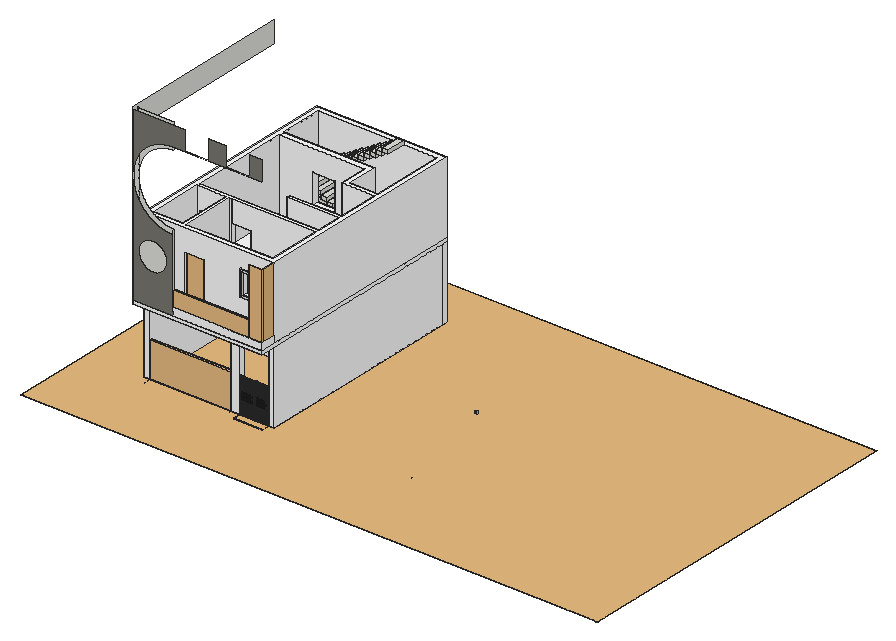
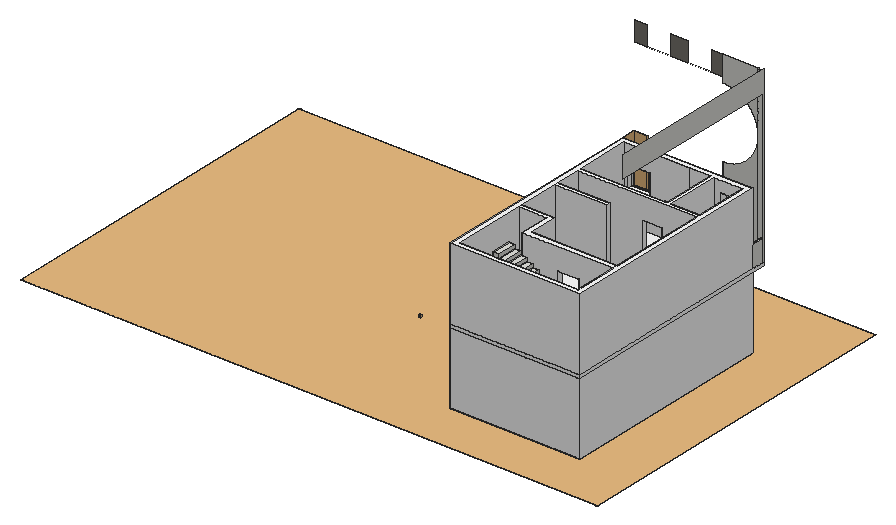
# SketchUp Ruby script. Lengths in inches.
U = 1.inch
M = Sketchup.active_model
def pt(a) = Geom::Point3d.new(a.map { |v| v * U })
def face(e, loops, mat)
  f = e.add_face(loops[0].map { |a| pt(a) })
  loops[1..].each { |l| e.add_face(l.map { |a| pt(a) }).erase! }
  f.material = f.back_material = mat if mat
  f
end
# faces: each face lists its corners as indices into pts; further lists are holes
def faces(e, pts, list, mat = nil) = list.each { |f| face(e, (f[0].is_a?(Array) ? f : [f]).map { |l| l.map { |i| pts[i] } }, mat) }
# xy, xz, yz: faces in a plane at the given z, y or x. An outline is a flat list of corners, or four numbers for a rectangle; further outlines are holes
def ring(l) = l.size == 4 ? [[l[0], l[1]], [l[2], l[1]], [l[2], l[3]], [l[0], l[3]]] : l.each_slice(2).to_a
def flat(e, list, mat, &to3) = list.each { |f| face(e, (f[0].is_a?(Array) ? f : [f]).map { |l| ring(l).map { |u, v| to3.(u, v) } }, mat) }
def xy(e, z, list, mat = nil) = flat(e, list, mat) { |x, y| [x, y, z] }
def xz(e, y, list, mat = nil) = flat(e, list, mat) { |x, z| [x, y, z] }
def yz(e, x, list, mat = nil) = flat(e, list, mat) { |y, z| [x, y, z] }
def lines(e, pts, list) = list.each { |a, b| e.add_line(pt(pts[a]), pt(pts[b])) }
# prism: a flat outline (further loops are holes) pulled along v
def prism(e, loops, v, mat = nil)
  f = face(e, loops, mat); d = Geom::Vector3d.new(v.map { |x| x * U })
  f.pushpull(f.normal.samedirection?(d) ? d.length : -d.length)
end
def box(e, o, s, mat = nil) = prism(e, [[o, [o[0] + s[0], o[1], o[2]], [o[0] + s[0], o[1] + s[1], o[2]], [o[0], o[1] + s[1], o[2]]]], [0, 0, s[2]], mat)
def at(x, y, z, deg = 0) = Geom::Transformation.translation(pt([x, y, z])) * Geom::Transformation.rotation(ORIGIN, Z_AXIS, deg.degrees)
def axes(o, x, y, z) = Geom::Transformation.new([*x, 0, *y, 0, *z, 0, *pt(o).to_a, 1])
def part(name) = M.definitions.add(name)
# library, detail: a bought-in or finely detailed component or shape, given as its bounding box
def library(name, o, s) = part(name).tap { |d| box(d.entities, o, s) }
def detail(e, o, s) = box(e.add_group.entities, o, s)
def put(e, d, t, mat = nil) = e.add_instance(d, t).tap { |i| i.material = mat if mat }
def group(e, t, mat = nil) = e.add_group.tap { |g| g.transformation = t; g.material = mat if mat }.entities
root = M.entities
M.materials.add("Color_008").color = [30, 30, 30]
M.materials.add("Manhattan Creative Coating ML 1016B 24.75cm").color = [255, 255, 255]
M.materials.add("Napura - nsi3013 29.32cm").color = [255, 255, 255]
M.materials.add("Sand Yellow 02 100cm").color = [219, 192, 169]
M.materials.add("Tiles L02 200cm").color = [152, 144, 134]
M.materials.add("[0055_LightGoldenrodYellow]").color = [250, 250, 210]
M.materials.add("[0131_Silver]").color = [192, 192, 192]
M.materials.add("[0134_DimGray]").color = [105, 105, 105]
M.materials.add("[Rough Square Concrete Block]").color = [123, 120, 113]
c1 = library("Garage Gate 243 111",[-105.76,-3.7,0],[211.52,7.4,101.23])
c2 = part("Screen slat")
box(c2.entities,[0,0,-2.03],[1.97,0.97,40.94])
c3 = part("Screen frame stile")
box(c3.entities,[0,0,0],[1.9,0.97,93.54])
c4 = part("Screen bar")
box(c4.entities,[2.95,0,-2.03],[0.99,0.97,40.94])
c5 = part("Slatted screen panel")
p = [[42.85,0.97,43.31],[42.85,0.97,44.29]]
lines(c5.entities,p,[[0,1]])
put(c5.entities,c2,axes([3.9375,0,86.61],[0,0,-1],[0,1,0],[1,0,0]),"Color_008")
put(c5.entities,c3,axes([87.6,0,0],[1,0,0],[0,1,0],[0,0,0.92593]),"Color_008")
put(c5.entities,c2,axes([48.6875,0,86.61],[0,0,-1],[0,1,0],[1,0,0]),"Color_008")
put(c5.entities,c3,axes([0,0,0],[1,0,0],[0,1,0],[0,0,0.92593]),"Color_008")
put(c5.entities,c3,axes([42.85,0,0],[1,0,0],[0,1,0],[0,0,0.92593]),"Color_008")
put(c5.entities,c3,axes([44.75,0,0],[1,0,0],[0,1,0],[0,0,0.92593]),"Color_008")
put(c5.entities,c4,axes([3.9375,0,87.11],[0,0,-1],[0,1,0],[1,0,0]),"[0134_DimGray]")
put(c5.entities,c4,axes([48.6875,0,87.11],[0,0,-1],[0,1,0],[1,0,0]),"[0134_DimGray]")
put(c5.entities,c2,axes([48.6875,0,82.68],[0,0,-1],[0,1,0],[1,0,0]),"Color_008")
put(c5.entities,c4,axes([48.6875,0,83.17],[0,0,-1],[0,1,0],[1,0,0]),"[0134_DimGray]")
put(c5.entities,c4,axes([3.9375,0,83.17],[0,0,-1],[0,1,0],[1,0,0]),"[0134_DimGray]")
put(c5.entities,c2,axes([3.9375,0,82.68],[0,0,-1],[0,1,0],[1,0,0]),"Color_008")
put(c5.entities,c4,axes([48.6875,0,75.3],[0,0,-1],[0,1,0],[1,0,0]),"[0134_DimGray]")
put(c5.entities,c2,axes([48.6875,0,78.74],[0,0,-1],[0,1,0],[1,0,0]),"Color_008")
put(c5.entities,c2,axes([48.6875,0,74.8],[0,0,-1],[0,1,0],[1,0,0]),"Color_008")
put(c5.entities,c4,axes([48.6875,0,79.23],[0,0,-1],[0,1,0],[1,0,0]),"[0134_DimGray]")
put(c5.entities,c4,axes([3.9375,0,75.3],[0,0,-1],[0,1,0],[1,0,0]),"[0134_DimGray]")
put(c5.entities,c2,axes([3.9375,0,78.74],[0,0,-1],[0,1,0],[1,0,0]),"Color_008")
put(c5.entities,c4,axes([3.9375,0,79.23],[0,0,-1],[0,1,0],[1,0,0]),"[0134_DimGray]")
put(c5.entities,c2,axes([3.9375,0,74.8],[0,0,-1],[0,1,0],[1,0,0]),"Color_008")
put(c5.entities,c4,axes([48.6875,0,67.42],[0,0,-1],[0,1,0],[1,0,0]),"[0134_DimGray]")
put(c5.entities,c4,axes([3.9375,0,63.48],[0,0,-1],[0,1,0],[1,0,0]),"[0134_DimGray]")
put(c5.entities,c4,axes([48.6875,0,71.36],[0,0,-1],[0,1,0],[1,0,0]),"[0134_DimGray]")
put(c5.entities,c4,axes([3.9375,0,67.42],[0,0,-1],[0,1,0],[1,0,0]),"[0134_DimGray]")
put(c5.entities,c2,axes([3.9375,0,70.87],[0,0,-1],[0,1,0],[1,0,0]),"Color_008")
put(c5.entities,c2,axes([48.6875,0,70.87],[0,0,-1],[0,1,0],[1,0,0]),"Color_008")
put(c5.entities,c2,axes([48.6875,0,66.93],[0,0,-1],[0,1,0],[1,0,0]),"Color_008")
put(c5.entities,c2,axes([48.6875,0,59.06],[0,0,-1],[0,1,0],[1,0,0]),"Color_008")
put(c5.entities,c2,axes([3.9375,0,55.12],[0,0,-1],[0,1,0],[1,0,0]),"Color_008")
put(c5.entities,c2,axes([3.9375,0,62.99],[0,0,-1],[0,1,0],[1,0,0]),"Color_008")
put(c5.entities,c4,axes([3.9375,0,59.55],[0,0,-1],[0,1,0],[1,0,0]),"[0134_DimGray]")
put(c5.entities,c2,axes([3.9375,0,66.93],[0,0,-1],[0,1,0],[1,0,0]),"Color_008")
put(c5.entities,c2,axes([48.6875,0,62.99],[0,0,-1],[0,1,0],[1,0,0]),"Color_008")
put(c5.entities,c4,axes([48.6875,0,59.55],[0,0,-1],[0,1,0],[1,0,0]),"[0134_DimGray]")
put(c5.entities,c4,axes([48.6875,0,63.48],[0,0,-1],[0,1,0],[1,0,0]),"[0134_DimGray]")
put(c5.entities,c2,axes([3.9375,0,59.06],[0,0,-1],[0,1,0],[1,0,0]),"Color_008")
put(c5.entities,c4,axes([3.9375,0,71.36],[0,0,-1],[0,1,0],[1,0,0]),"[0134_DimGray]")
put(c5.entities,c4,axes([3.9375,0,33.96],[0,0,-1],[0,1,0],[1,0,0]),"[0134_DimGray]")
put(c5.entities,c4,axes([48.6875,0,33.96],[0,0,-1],[0,1,0],[1,0,0]),"[0134_DimGray]")
put(c5.entities,c2,axes([3.9375,0,29.53],[0,0,-1],[0,1,0],[1,0,0]),"Color_008")
put(c5.entities,c4,axes([3.9375,0,26.08],[0,0,-1],[0,1,0],[1,0,0]),"[0134_DimGray]")
put(c5.entities,c2,axes([3.9375,0,33.46],[0,0,-1],[0,1,0],[1,0,0]),"Color_008")
put(c5.entities,c2,axes([48.6875,0,29.53],[0,0,-1],[0,1,0],[1,0,0]),"Color_008")
put(c5.entities,c4,axes([48.6875,0,30.02],[0,0,-1],[0,1,0],[1,0,0]),"[0134_DimGray]")
put(c5.entities,c2,axes([3.9375,0,25.59],[0,0,-1],[0,1,0],[1,0,0]),"Color_008")
put(c5.entities,c2,axes([48.6875,0,25.59],[0,0,-1],[0,1,0],[1,0,0]),"Color_008")
put(c5.entities,c2,axes([48.6875,0,33.46],[0,0,-1],[0,1,0],[1,0,0]),"Color_008")
put(c5.entities,c2,axes([3.9375,0,49.7],[0,0,-1],[0,1,0],[1,0,0]),"Color_008")
put(c5.entities,c4,axes([48.6875,0,26.08],[0,0,-1],[0,1,0],[1,0,0]),"[0134_DimGray]")
put(c5.entities,c4,axes([3.9375,0,30.02],[0,0,-1],[0,1,0],[1,0,0]),"[0134_DimGray]")
put(c5.entities,c2,axes([3.9375,0,5.91],[0,0,-1],[0,1,0],[1,0,0]),"Color_008")
put(c5.entities,c2,axes([48.6875,0,13.78],[0,0,-1],[0,1,0],[1,0,0]),"Color_008")
put(c5.entities,c4,axes([48.6875,0,10.33],[0,0,-1],[0,1,0],[1,0,0]),"[0134_DimGray]")
put(c5.entities,c4,axes([3.9375,0,6.4],[0,0,-1],[0,1,0],[1,0,0]),"[0134_DimGray]")
put(c5.entities,c2,axes([3.9375,0,13.78],[0,0,-1],[0,1,0],[1,0,0]),"Color_008")
put(c5.entities,c2,axes([48.6875,0,21.65],[0,0,-1],[0,1,0],[1,0,0]),"Color_008")
put(c5.entities,c2,axes([48.6875,0,5.91],[0,0,-1],[0,1,0],[1,0,0]),"Color_008")
put(c5.entities,c4,axes([48.6875,0,22.15],[0,0,-1],[0,1,0],[1,0,0]),"[0134_DimGray]")
put(c5.entities,c2,axes([48.6875,0,1.97],[0,0,-1],[0,1,0],[1,0,0]),"Color_008")
put(c5.entities,c2,axes([48.6875,0,9.84],[0,0,-1],[0,1,0],[1,0,0]),"Color_008")
put(c5.entities,c4,axes([48.6875,0,6.4],[0,0,-1],[0,1,0],[1,0,0]),"[0134_DimGray]")
put(c5.entities,c2,axes([3.9375,0,9.84],[0,0,-1],[0,1,0],[1,0,0]),"Color_008")
put(c5.entities,c4,axes([3.9375,0,10.33],[0,0,-1],[0,1,0],[1,0,0]),"[0134_DimGray]")
put(c5.entities,c4,axes([3.9375,0,22.15],[0,0,-1],[0,1,0],[1,0,0]),"[0134_DimGray]")
put(c5.entities,c2,axes([3.9375,0,1.97],[0,0,-1],[0,1,0],[1,0,0]),"Color_008")
put(c5.entities,c4,axes([3.9375,0,18.21],[0,0,-1],[0,1,0],[1,0,0]),"[0134_DimGray]")
put(c5.entities,c4,axes([3.9375,0,14.27],[0,0,-1],[0,1,0],[1,0,0]),"[0134_DimGray]")
put(c5.entities,c2,axes([3.9375,0,21.65],[0,0,-1],[0,1,0],[1,0,0]),"Color_008")
put(c5.entities,c4,axes([48.6875,0,18.21],[0,0,-1],[0,1,0],[1,0,0]),"[0134_DimGray]")
put(c5.entities,c2,axes([3.9375,0,17.72],[0,0,-1],[0,1,0],[1,0,0]),"Color_008")
put(c5.entities,c2,axes([48.6875,0,17.72],[0,0,-1],[0,1,0],[1,0,0]),"Color_008")
put(c5.entities,c4,axes([48.6875,0,14.27],[0,0,-1],[0,1,0],[1,0,0]),"[0134_DimGray]")
put(c5.entities,c2,axes([3.9375,0,44.29],[0,0,-1],[0,1,0],[1,0,0]),"Color_008")
put(c5.entities,c2,axes([3.9375,0,38.88],[0,0,-1],[0,1,0],[1,0,0]),"Color_008")
put(c5.entities,c2,axes([48.6875,0,49.7],[0,0,-1],[0,1,0],[1,0,0]),"Color_008")
put(c5.entities,c2,axes([48.6875,0,44.29],[0,0,-1],[0,1,0],[1,0,0]),"Color_008")
put(c5.entities,c2,axes([48.6875,0,38.88],[0,0,-1],[0,1,0],[1,0,0]),"Color_008")
put(c5.entities,c2,axes([48.6875,0,55.12],[0,0,-1],[0,1,0],[1,0,0]),"Color_008")
c6 = part("Infill panel")
box(c6.entities,[0,0,-9.84],[39.64,0.39,36.58])
c7 = part("Infill panel \#1")
box(c7.entities,[0,0,-1.97],[52.81,0.39,23.62])
c8 = library("PLAN 2.dwg",[89.6,971.62,0],[961.37,580.64,0.01])
c9 = part("Stair tread")
box(c9.entities,[0,0,0],[10,33,6])
c10 = part("Stair landing")
box(c10.entities,[-32,0,0],[42,72,6])
c11 = part("Group\#2")
put(c11.entities,c9,at(82,39,90))
put(c11.entities,c9,at(92,39,96))
put(c11.entities,c9,at(102,39,102))
put(c11.entities,c9,at(72,39,84))
put(c11.entities,c9,at(112,39,108))
put(c11.entities,c9,at(62,39,78))
put(c11.entities,c9,at(122,39,114))
put(c11.entities,c9,at(52,39,72))
put(c11.entities,c9,at(52,0,48))
put(c11.entities,c9,at(42,0,54))
put(c11.entities,c10,at(32,0,60))
put(c11.entities,c9,at(112,0,12))
put(c11.entities,c9,at(122,0,6))
put(c11.entities,c9,at(82,0,30))
put(c11.entities,c9,at(92,0,24))
put(c11.entities,c9,at(72,0,36))
put(c11.entities,c9,at(62,0,42))
put(c11.entities,c9,at(132,0,0))
put(c11.entities,c9,at(102,0,18))
put(c11.entities,c9,at(42,39,66))
put(c11.entities,c9,at(132,39,120))
c12 = library("Window Crafter Sliding 3",[0,-0.55,0],[36,4.49,48])
c13 = library("Door 243 053",[-21.6,-2.79,-0.07],[43.2,5.58,82.64])
c14 = part("Group\#14")
box(c14.entities,[0,0,0],[3,21,36])
c15 = library("Group\#12",[0,0,0],[21.6875,1,109.4375])
c16 = library("Group\#18",[0,0,0],[21.6875,1,109.4375])
c17 = library("Group\#15",[0,0,0],[131.45,3.15,25.98])
xy(root,-18.0625,[[9.02,62.93,144,74.93]])
xy(root,0,[[439.05,74.93,475.05,83.93]])
xy(root,0,[[144,74.93,159,83.93]],"Manhattan Creative Coating ML 1016B 24.75cm")
xy(root,120,[[144,74.93,159,83.93]],"Manhattan Creative Coating ML 1016B 24.75cm")
xy(root,126,[[0,50.93,0,53.93,213,53.93,213,74.93,216,74.93,216,50.93]])
xy(root,138,[[66.79,50.93,216,50.93,216,74.93,213,74.93,213,53.93,66.79,53.93]])
xz(root,50.93,[[66.79,126,216,138]],"Manhattan Creative Coating ML 1016B 24.75cm")
xz(root,50.93,[[[0,126,66.79,126,66.79,246,65.41,246.01,64.03,246.06,62.65,246.13,61.27,246.23,59.9,246.36,58.52,246.52,57.15,246.71,55.79,246.92,54.43,247.17,53.07,247.44,51.72,247.74,50.38,248.07,49.05,248.43,47.72,248.82,46.4,249.23,45.09,249.67,43.79,250.14,42.5,250.63,41.22,251.16,39.95,251.71,38.69,252.28,37.45,252.88,36.22,253.51,35,254.16,33.79,254.84,32.61,255.55,31.43,256.27,30.27,257.03,29.13,257.8,28,258.6,26.89,259.43,25.8,260.28,24.72,261.15,23.67,262.04,22.63,262.95,21.61,263.89,20.62,264.84,19.64,265.82,18.68,266.82,17.75,267.84,16.83,268.875,15.94,269.93,15.07,271,14.22,272.1,13.4,273.21,12.6,274.33,11.82,275.48,11.07,276.64,10.34,277.81,9.64,279,8.96,280.2,8.31,281.42,7.68,282.65,7.08,283.9,6.5,285.16,5.95,286.42,5.43,287.7,4.93,288.99,4.47,290.29,4.03,291.6,3.61,292.92,3.23,294.25,2.87,295.59,2.54,296.93,2.24,298.28,1.96,299.63,1.72,300.99,1.5,302.36,1.32,303.73,1.16,305.1,1.03,306.48,0.93,307.86,0.85,309.24,0.81,310.62,0.79,312,0.81,313.38,0.85,314.76,0.93,316.14,1.03,317.52,1.16,318.9,1.32,320.27,1.5,321.64,1.72,323.01,1.96,324.37,2.24,325.72,2.54,327.07,2.87,328.41,3.23,329.75,3.61,331.08,4.03,332.4,4.47,333.71,4.93,335.01,5.43,336.3,5.95,337.58,6.5,338.84,7.08,340.1,7.68,341.35,8.31,342.58,8.96,343.8,9.64,345,10.34,346.19,11.07,347.36,11.82,348.52,12.6,349.67,13.4,350.79,14.22,351.9,15.07,353,15.94,354.07,16.83,355.125,17.75,356.16,18.68,357.18,19.64,358.18,20.62,359.16,21.61,360.11,22.63,361.05,23.67,361.96,24.72,362.85,25.8,363.72,26.89,364.57,28,365.4,29.13,366.2,30.27,366.97,31.43,367.73,32.61,368.45,33.79,369.16,35,369.84,36.22,370.49,37.45,371.12,38.69,371.72,39.95,372.29,41.22,372.84,42.5,373.37,43.79,373.86,45.09,374.33,46.4,374.77,47.72,375.18,49.05,375.57,50.38,375.93,51.72,376.26,53.07,376.56,54.43,376.83,55.79,377.08,57.15,377.29,58.52,377.48,59.9,377.64,61.27,377.77,62.65,377.87,64.03,377.94,65.41,377.99,66.79,378,216,378,216,410.75,195.25,410.75,195.25,378.5,155.15,378.5,155.15,410.75,127.65,410.75,127.65,378.5,87.54,378.5,87.54,410.75,0,410.75],[33.9,178.41,32.91,178.42,31.91,178.48,30.92,178.58,29.9375,178.72,28.96,178.9,27.99,179.12,27.03,179.38,26.08,179.6875,25.15,180.03,24.23,180.41,23.33,180.83,22.44,181.28,21.58,181.78,20.74,182.31,19.92,182.87,19.12,183.47,18.35,184.1,17.61,184.76,16.89,185.45,16.21,186.17,15.56,186.92,14.93,187.7,14.35,188.5,13.79,189.33,13.27,190.17,12.79,191.04,12.34,191.93,11.93,192.84,11.56,193.76,11.23,194.7,10.9375,195.65,10.68,196.61,10.47,197.59,10.3,198.57,10.17,199.55,10.08,200.54,10.04,201.54,10.03,202.53,10.07,203.52,10.15,204.52,10.27,205.5,10.43,206.49,10.63,207.46,10.87,208.42,11.15,209.38,11.48,210.32,11.84,211.25,12.24,212.16,12.67,213.05,13.15,213.92,13.66,214.78,14.21,215.61,14.79,216.42,15.4,217.2,16.05,217.96,16.72,218.68,17.43,219.38,18.17,220.05,18.93,220.69,19.72,221.3,20.53,221.87,21.37,222.41,22.23,222.91,23.11,223.375,24.01,223.8,24.92,224.19,25.85,224.54,26.8,224.86,27.75,225.13,28.72,225.36,29.7,225.55,30.68,225.7,31.67,225.8125,32.66,225.88,33.66,225.91,34.65,225.89,35.64,225.83,36.63,225.73,37.62,225.59,38.6,225.41,39.57,225.1875,40.53,224.93,41.47,224.625,42.41,224.28,43.33,223.9,44.23,223.48,45.11,223.03,45.98,222.53,46.82,222,47.64,221.44,48.43,220.84,49.2,220.21,49.95,219.55,50.66,218.86,51.35,218.14,52,217.39,52.62,216.61,53.21,215.81,53.77,214.98,54.28,214.14,54.77,213.27,55.22,212.38,55.625,211.47,56,210.55,56.33,209.61,56.62,208.66,56.87,207.7,57.08,206.73,57.25,205.75,57.38,204.76,57.47,203.77,57.52,202.77,57.52,201.78,57.49,200.79,57.41,199.79,57.29,198.81,57.13,197.82,56.93,196.85,56.69,195.89,56.4,194.93,56.08,193.99,55.72,193.0625,55.32,192.15,54.88,191.26,54.41,190.39,53.9,189.53,53.35,188.7,52.77,187.89,52.16,187.11,51.51,186.35,50.83,185.625,50.125,184.93,49.39,184.26,48.625,183.62,47.84,183.01,47.02,182.44,46.19,181.9,45.33,181.4,44.45,180.9375,43.55,180.51,42.63,180.12,41.7,179.77,40.76,179.45,39.8,179.18,38.84,178.95,37.86,178.76,36.875,178.61,35.89,178.5,34.89,178.43]]],"[Rough Square Concrete Block]")
xz(root,53.93,[[0,126,0,378,6,378,6,414,7.1875,414,7.1875,126],[7.1875,126,7.1875,414,66.79,414,66.79,371.45,65.55,371.44,64.31,371.4,63.0625,371.33,61.82,371.24,60.58,371.12,59.34,370.98,58.11,370.8125,56.88,370.62,55.66,370.4,54.43,370.15,53.22,369.88,52.01,369.58,50.81,369.26,49.61,368.91,48.42,368.54,47.24,368.14,46.07,367.72,44.91,367.27,43.76,366.8,42.62,366.31,41.48,365.79,40.36,365.25,39.25,364.68,38.16,364.1,37.07,363.48,36,362.85,34.94,362.19,33.9,361.52,32.87,360.82,31.85,360.09,30.85,359.35,29.87,358.59,28.9,357.81,27.95,357,27.02,356.18,26.1,355.34,25.2,354.47,24.32,353.59,23.46,352.7,22.62,351.78,21.79,350.84,20.99,349.89,20.21,348.93,19.44,347.94,18.7,346.94,17.98,345.93,17.28,344.9,16.6,343.85,15.94,342.8,15.3125,341.72,14.7,340.64,14.11,339.54,13.55,338.43,13,337.3125,12.49,336.18,11.99,335.04,11.52,333.88,11.07,332.72,10.65,331.55,10.26,330.37,9.88,329.18,9.54,327.99,9.21,326.78,8.92,325.58,8.65,324.36,8.4,323.14,8.18,321.91,7.98,320.68,7.82,319.45,7.67,318.21,7.55,316.97,7.46,315.73,7.4,314.49,7.36,313.24,7.35,312,7.36,310.76,7.4,309.51,7.46,308.27,7.55,307.03,7.67,305.79,7.82,304.55,7.98,303.32,8.18,302.09,8.4,300.86,8.65,299.64,8.92,298.42,9.21,297.22,9.54,296.01,9.88,294.82,10.26,293.63,10.65,292.45,11.07,291.28,11.52,290.12,11.99,288.96,12.49,287.82,13,286.6875,13.55,285.57,14.11,284.46,14.7,283.36,15.3125,282.28,15.94,281.2,16.6,280.15,17.28,279.1,17.98,278.07,18.7,277.06,19.44,276.06,20.21,275.07,20.99,274.11,21.79,273.16,22.62,272.22,23.46,271.3,24.32,270.41,25.2,269.53,26.1,268.66,27.02,267.82,27.95,267,28.9,266.19,29.87,265.41,30.85,264.65,31.85,263.91,32.87,263.18,33.9,262.48,34.94,261.81,36,261.15,37.07,260.52,38.16,259.9,39.25,259.32,40.36,258.75,41.48,258.21,42.62,257.69,43.76,257.2,44.91,256.73,46.07,256.28,47.24,255.86,48.42,255.46,49.61,255.09,50.81,254.74,52.01,254.42,53.22,254.12,54.43,253.85,55.66,253.6,56.88,253.38,58.11,253.1875,59.34,253.02,60.58,252.88,61.82,252.76,63.0625,252.67,64.31,252.6,65.55,252.56,66.79,252.55,66.79,138,213,138,213,126]])
xz(root,74.93,[[9.02,-18.0625,144,0],[213,126,216,138]])
xz(root,74.93,[[144,0,159,120]],"Manhattan Creative Coating ML 1016B 24.75cm")
xz(root,83.93,[[144,0,159,120]],"Manhattan Creative Coating ML 1016B 24.75cm")
yz(root,0,[[50.93,126,50.93,414,344.93,414,344.93,378,53.93,378,53.93,126]])
yz(root,9.02,[[62.93,-18.0625,0,-12.68,74.93,0,74.93,-18.0625]],"Tiles L02 200cm")
yz(root,66.79,[[50.93,138,53.93,252]])
yz(root,144,[[74.93,0,83.93,120]],"Manhattan Creative Coating ML 1016B 24.75cm")
yz(root,144,[[62.93,-18.0625,74.93,-18.0625,74.93,0,0,-12.68]],"Tiles L02 200cm")
yz(root,159,[[74.93,0,83.93,120]],"Manhattan Creative Coating ML 1016B 24.75cm")
yz(root,213,[[53.93,126,74.93,138]])
yz(root,216,[[50.93,126,74.93,138]],"Manhattan Creative Coating ML 1016B 24.75cm")
p = [[144,62.93,-18.0625],[144,0,-12.68],[9.02,0,-12.68],[9.02,62.93,-18.0625],[144,74.93,0],[9.02,74.93,0]]
faces(root,p,[[0,1,2,3]])
faces(root,p,[[4,5,2,1]],"Tiles L02 200cm")
detail(root,[396.17,269.2,0],[3.35,1.53,3.25])
g1 = group(root,at(0,74.93,-6),"Sand Yellow 02 100cm")
box(g1,[0,0,-12.0625],[216,360,18.0625])
g2 = group(root,at(158.95,38.93,-18),"Tiles L02 200cm")
prism(g2,[[[48,-1,5.57],[48,-1,5.5],[48,-1,5.43],[48,-0.98,5.37],[48,-0.96,5.31],[48,-0.93,5.25],[48,-0.9,5.2],[48,-0.85,5.15],[48,-0.8,5.1],[48,-0.75,5.07],[48,-0.69,5.04],[48,-0.63,5.02],[48,-0.57,5],[48,-0.5,5],[48,0,5],[48,0,0],[48,36,0],[48,36,6],[48,-0.5,6],[48,-0.57,6],[48,-0.63,5.98],[48,-0.69,5.96],[48,-0.75,5.93],[48,-0.8,5.9],[48,-0.85,5.85],[48,-0.9,5.8],[48,-0.93,5.75],[48,-0.96,5.69],[48,-0.98,5.63]]],[-48,0,0])
g3 = group(root,at(158.97,50.93,-12),"Tiles L02 200cm")
prism(g3,[[[48,-1,5.57],[48,-1,5.5],[48,-1,5.43],[48,-0.98,5.37],[48,-0.96,5.31],[48,-0.93,5.25],[48,-0.9,5.2],[48,-0.85,5.15],[48,-0.8,5.1],[48,-0.75,5.07],[48,-0.69,5.04],[48,-0.63,5.02],[48,-0.57,5],[48,-0.5,5],[48,0,5],[48,0,0],[48,24,0],[48,24,6],[48,-0.5,6],[48,-0.57,6],[48,-0.63,5.98],[48,-0.69,5.96],[48,-0.75,5.93],[48,-0.8,5.9],[48,-0.85,5.85],[48,-0.9,5.8],[48,-0.93,5.75],[48,-0.96,5.69],[48,-0.98,5.63]]],[-48,0,0])
g4 = group(root,at(159,62.93,-6),"Tiles L02 200cm")
prism(g4,[[[48,-1,5.57],[48,-1,5.5],[48,-1,5.43],[48,-0.98,5.37],[48,-0.96,5.31],[48,-0.93,5.25],[48,-0.9,5.2],[48,-0.85,5.15],[48,-0.8,5.1],[48,-0.75,5.07],[48,-0.69,5.04],[48,-0.63,5.02],[48,-0.57,5],[48,-0.5,5],[48,0,5],[48,0,0],[48,12,0],[48,12,6],[48,-0.5,6],[48,-0.57,6],[48,-0.63,5.98],[48,-0.69,5.96],[48,-0.75,5.93],[48,-0.8,5.9],[48,-0.85,5.85],[48,-0.9,5.8],[48,-0.93,5.75],[48,-0.96,5.69],[48,-0.98,5.63]]],[-48,0,0])
put(root,c1,axes([76.51,77.08,-0.01],[0.6383,0,0],[0,0.58,0],[0,0,0.58]))
g5 = group(root,at(159,74.67,0))
put(g5,c5,axes([0,0.27,0],[0.5366,0,0],[0,0.6762,0],[0,0,0.6762]),"[0055_LightGoldenrodYellow]")
put(g5,c6,axes([1.02,0.92,42.64],[0.58009,0,0],[0,0.6762,0],[0,0,0.54583]),"[0131_Silver]")
put(g5,c7,axes([0,0,22.63],[0.45474,0,0],[0,0.6762,0],[0,0,0.6762]),"Color_008")
put(g5,c7,axes([24.01,0,22.63],[0.45474,0,0],[0,0.6762,0],[0,0,0.6762]),"Color_008")
put(g5,c6,axes([24.01,0.92,42.64],[0.58009,0,0],[0,0.6762,0],[0,0,0.54583]),"[0131_Silver]")
put(g5,c6,axes([24.01,0.92,6.7],[0.58009,0,0],[0,0.6762,0],[0,0,0.54583]),"[0131_Silver]")
put(g5,c6,axes([1.02,0.92,6.7],[0.58009,0,0],[0,0.6762,0],[0,0,0.54583]),"[0131_Silver]")
put(root,c8,at(-185.17,-1035.07,0))
g6 = group(root,at(0,74.93,0))
xy(g6,0,[[160.92,144,161,228.1]])
xy(g6,36,[[51,144,87,153]],"Napura - nsi3013 29.32cm")
xy(g6,84,[[152,228.1,161,264.1]])
xy(g6,84,[[51,144,87,153]],"Napura - nsi3013 29.32cm")
xy(g6,120,[[0,0,9,0,9,270,152,270,152,153,9,153,9,144,161,144,161,279,9,279,9,351,216,351,216,360,0,360],[207,0,216,351]])
xz(g6,0,[[0,0,9,120],[207,0,216,120]],"Manhattan Creative Coating ML 1016B 24.75cm")
xz(g6,144,[[[9,0,161,120],[51,36,87,84]]],"Napura - nsi3013 29.32cm")
xz(g6,153,[[[9,0,152,120],[51,36,87,84]]])
xz(g6,228.1,[[152,0,161,84]])
xz(g6,264.1,[[152,0,161,84]])
xz(g6,270,[[9,0,152,120]])
xz(g6,279,[[9,0,161,120]])
xz(g6,351,[[9,0,207,120]])
xz(g6,360,[[0,0,216,120]],"Napura - nsi3013 29.32cm")
yz(g6,0,[[0,0,360,120]],"Napura - nsi3013 29.32cm")
yz(g6,9,[[153,0,270,120],[279,0,351,120]])
yz(g6,9,[[0,0,144,120]],"Napura - nsi3013 29.32cm")
yz(g6,51,[[144,36,153,84]],"Napura - nsi3013 29.32cm")
yz(g6,87,[[144,36,153,84]],"Napura - nsi3013 29.32cm")
yz(g6,152,[[153,0,153,120,264.1,120,264.1,84,228.1,84,228.1,0],[264.1,0,270,120]])
yz(g6,161,[[144,0,228.1,0,228.1,84,264.1,84,264.1,0,279,0,279,120,144,120]])
yz(g6,207,[[0,0,351,120]])
yz(g6,216,[[0,0,351,120],[351,0,360,120]],"Napura - nsi3013 29.32cm")
p = [[160.92,228.13,0],[160.92,228.1,0],[152,228.13,0],[152,228.1,0]]
lines(g6,p,[[0,1],[2,3],[2,0]])
put(root,c11,at(9,353.93,0))
put(root,c12,at(51,221.74,36))
g7 = group(root,at(0,74.93,120),"Manhattan Creative Coating ML 1016B 24.75cm")
prism(g7,[[[0,-24,0],[0,360,0],[216,360,0],[216,-24,0]],[[151,279,0],[151,351,0],[9,351,0],[9,279,0]]],[0,0,6])
put(root,c13,axes([83,82.09,125.85],[0.7407,0,0],[0,1,0],[0,0,1.02907]))
put(root,c11,at(9,353.93,126))
g8 = group(root,at(0,74.93,126),"Napura - nsi3013 29.32cm")
xy(g8,0,[[9,0,9,9,57,9,57,99,45.13,99,45.13,105,67.04,105,67.04,98.09,63,98.09,63,9,67,9,67,0],[9,99,13,105],[99,99,207,105],[120,147,207,153]])
xy(g8,36,[[65.47,270,101.47,279]])
xy(g8,54,[[164.22,0,200.22,9]])
xy(g8,84,[[21,0,45,9],[67,0,99,9],[13,99,45.13,105],[67.04,99,99,105],[152,228,161,263.99],
  [65.47,270,101.47,279]])
xy(g8,90,[[164.22,0,200.22,9]])
xy(g8,102,[[21,0,45,9]])
xy(g8,120,[[0,0,9,0,9,99,57,99,57,9,9,9,9,0,216,0,216,360,9,360,9,351,207,351,207,9,63,9,63,98.09,67.04,98.09,67.04,99,207,99,207,105,9,105,9,360,0,360],[120,147,207,153],[152,222,207,222,207,228,161,228,161,279,9,279,9,270,152,270]])
xz(g8,0,[[0,0,9,120]])
xz(g8,0,[[[9,0,67,0,67,84,99,84,99,0,216,0,216,120,9,120],[164.22,54,200.22,90],[21,84,45,102]]],"Napura - nsi3013 29.32cm")
xz(g8,9,[[[9,0,57,120],[21,84,45,102]],[63,0,63,120,99,120,99,84,67,84,67,0],[[99,0,207,120],[164.22,54,200.22,90]]])
xz(g8,98.09,[[63,0,67.04,120]])
xz(g8,99,[[9,0,13,0,13,84,45.13,84,45.13,0,57,0,57,120,9,120],[99,0,207,0,207,120,67.04,120,67.04,84,99,84]])
xz(g8,105,[[9,0,9,120,207,120,207,0,99,0,99,84,67.04,84,67.04,0,45.13,0,45.13,84,13,84,13,0]])
xz(g8,147,[[120,0,207,120]])
xz(g8,153,[[120,0,207,120]])
xz(g8,222,[[152,0,207,120]])
xz(g8,228,[[152,0,152,84,161,84,161,120,207,120,207,0]])
xz(g8,263.99,[[152,0,161,84]])
xz(g8,270,[[[9,0,152,120],[65.47,36,101.47,84]]])
xz(g8,279,[[[9,0,161,120],[65.47,36,101.47,84]]])
xz(g8,351,[[9,0,207,120]])
xz(g8,360,[[0,0,216,120]],"Napura - nsi3013 29.32cm")
yz(g8,0,[[0,0,360,120]],"Napura - nsi3013 29.32cm")
yz(g8,9,[[9,0,99,120],[105,0,270,120],[279,0,351,120]])
yz(g8,13,[[99,0,105,84]])
yz(g8,21,[[0,84,9,102]])
yz(g8,45,[[0,84,9,102]])
yz(g8,45.13,[[99,0,105,84]])
yz(g8,57,[[9,0,99,120]])
yz(g8,63,[[9,0,98.09,120]])
yz(g8,65.47,[[270,36,279,84]])
yz(g8,67,[[0,0,9,84]])
yz(g8,67.04,[[98.09,0,105,0,105,84,99,84,99,120,98.09,120]])
yz(g8,99,[[0,0,9,84],[99,0,105,84]])
yz(g8,101.47,[[270,36,279,84]])
yz(g8,120,[[147,0,153,120]])
yz(g8,152,[[222,0,222,120,270,120,270,0,263.99,0,263.99,84,228,84,228,0]])
yz(g8,161,[[263.99,0,279,0,279,120,228,120,228,84,263.99,84]])
yz(g8,164.22,[[0,54,9,90]])
yz(g8,200.22,[[0,54,9,90]])
yz(g8,207,[[9,0,99,120],[105,0,147,120],[153,0,222,120],[228,0,351,120]])
yz(g8,216,[[0,0,360,120]],"Napura - nsi3013 29.32cm")
put(root,c14,at(0,53.93,126))
put(root,c15,axes([194.3125,50.93,138],[1,0,0],[0,1,0],[0,0,0.98686]))
put(root,c16,axes([216,53.24,138],[0,1,0],[-1,0,0],[0,0,0.98686]))
put(root,c17,axes([66.79,50.93,138],[0.97005,0,0],[0,1,0],[0,0,1]))
g9 = group(root,at(161.22,72.93,177))
prism(g9,[[[42,2,0],[0,2,0],[0,2,42],[42,2,42]],[[39,2,39],[3,2,39],[3,2,3],[39,2,3]]],[0,-2,0])
